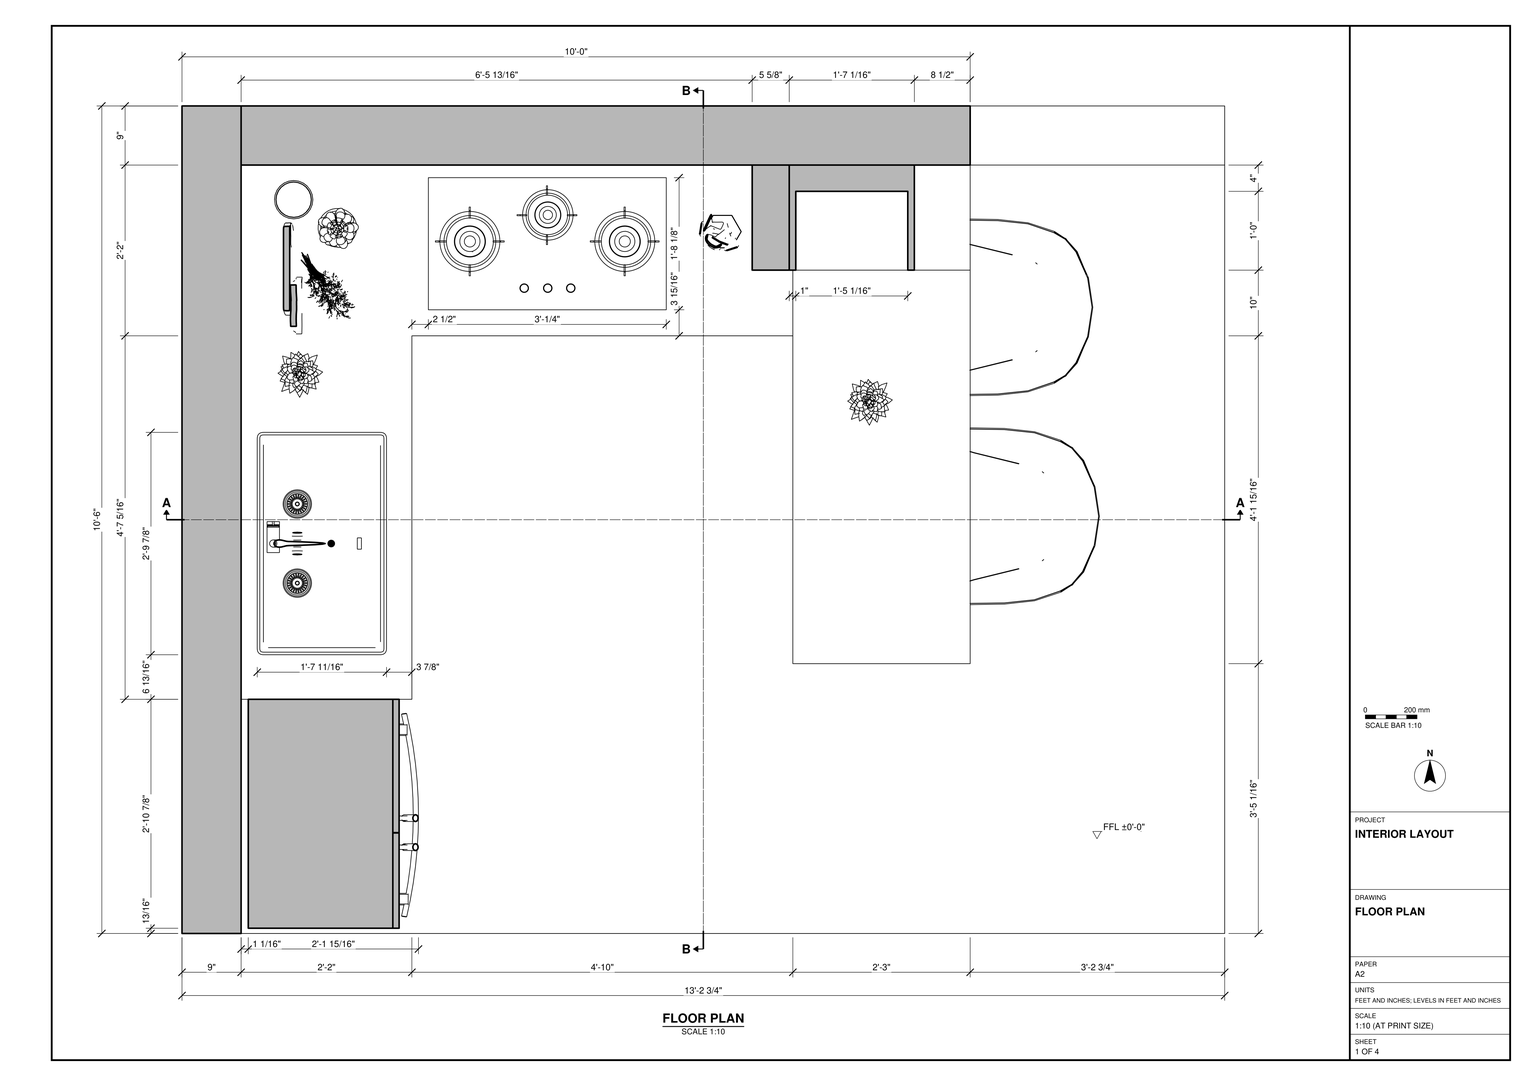
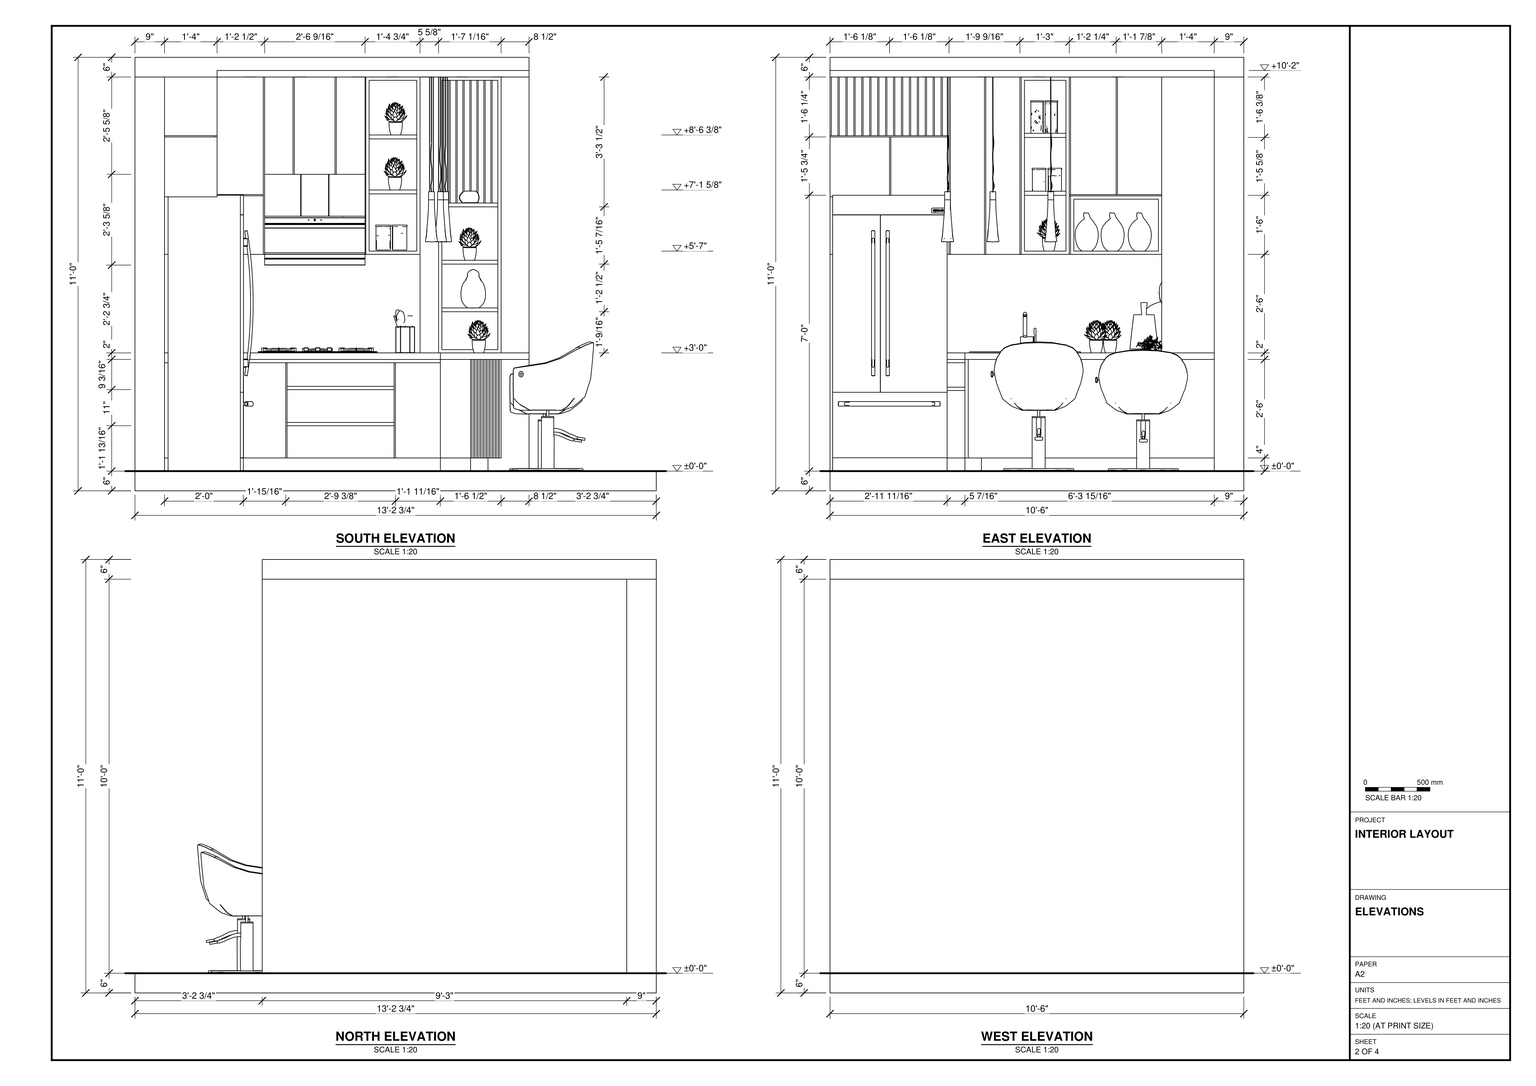
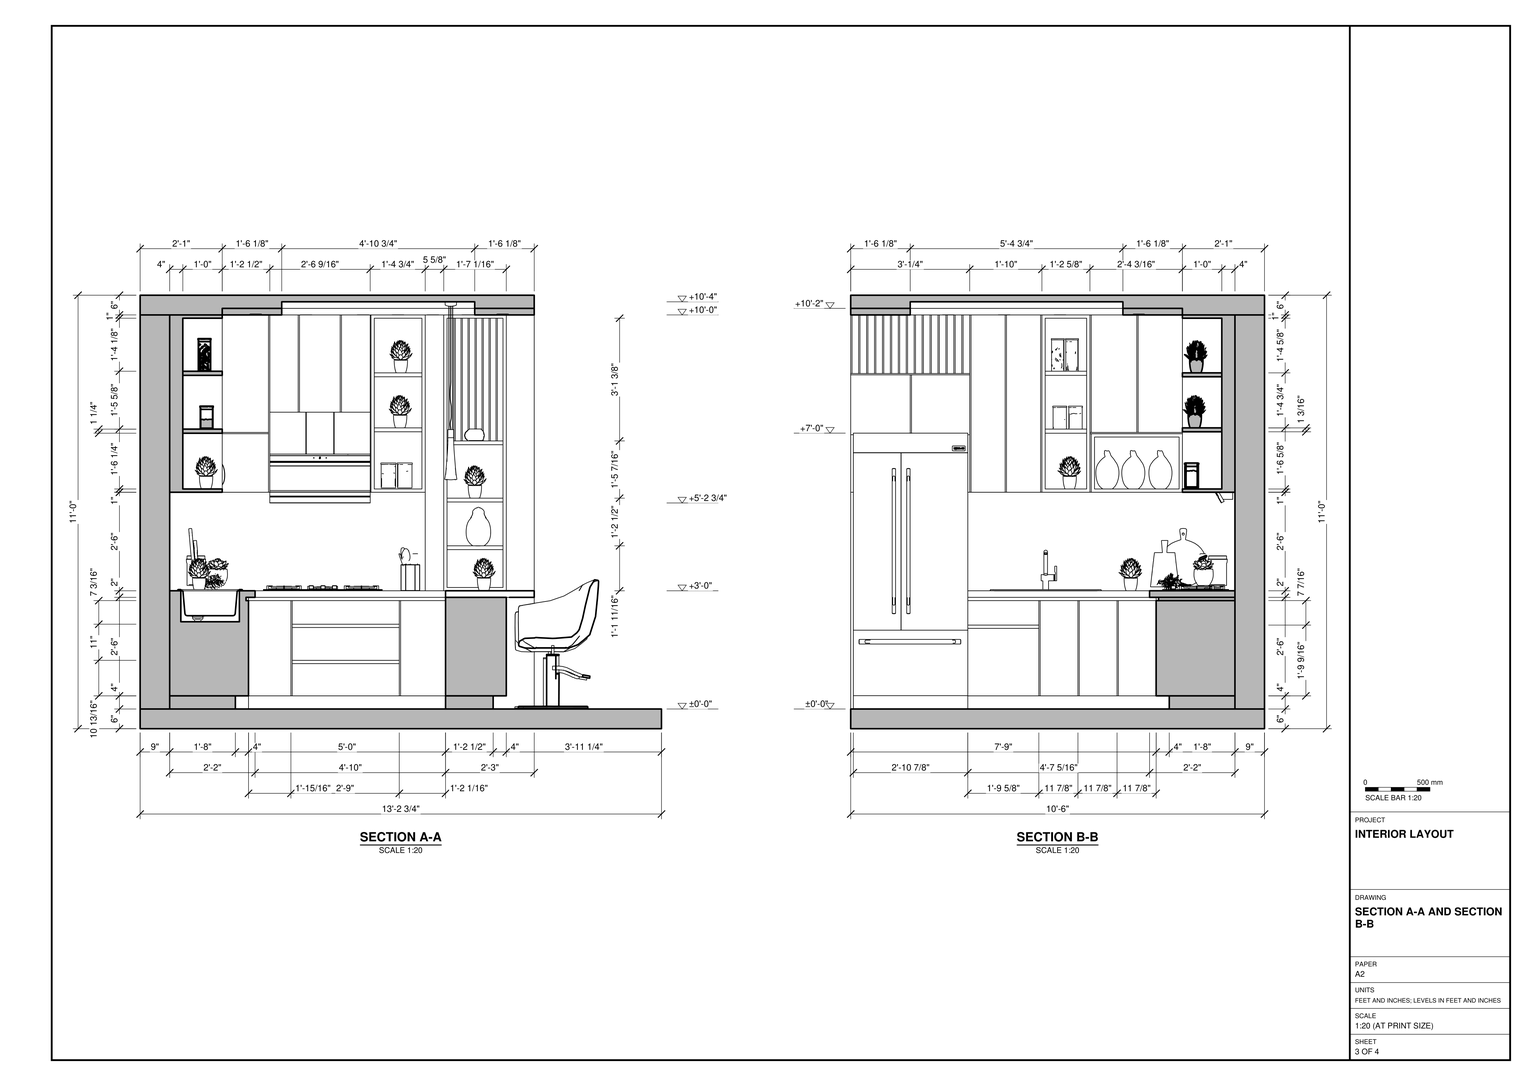
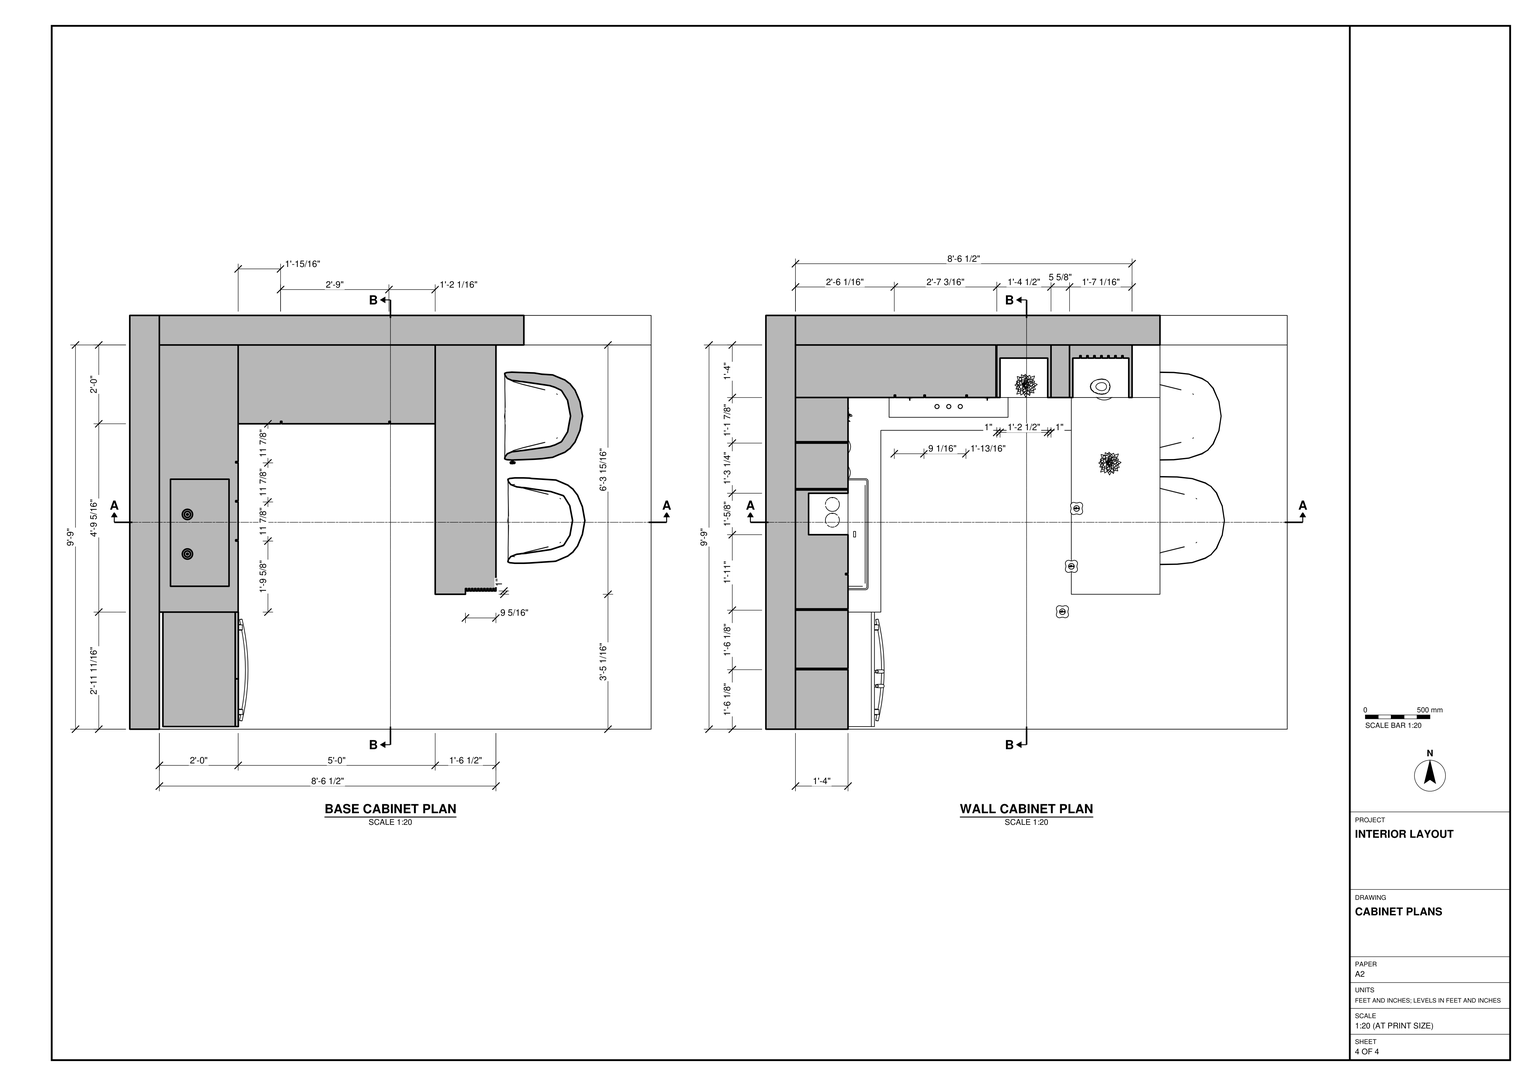
Build the kitchen interior in SketchUp from task_files/diagram_01.pdf. Work in feet and inches. The overall model measures 13'-2 3/4" along X, 10'-6" along Y and 11'-0" along Z. Set the finished floor at ±0'-0". Model the floor slab, the 9" thick north and west walls, and the stepped ceiling slab shown in section. The floor extends east beyond the end of the north wall to accommodate the seating.

Lay out the worktop along the two walls, with the sink and tap on the west run, the refrigerator at its south end, and the cooktop beneath the hood on the north run. Use the elevations and sections to set out the recessed plinths, base cabinet doors, drawer stack, upper cupboards, open shelves and vertically slatted panels. Match the shelf divisions around the hood and above the peninsula rather than treating the upper storage as a continuous bank of doors.

Project the peninsula south from the north run, leaving the working aisle between it and the sink. Place the two seats along its east edge and the pendant lights above it as drawn. Decor and loose items, including plants, vessels, utensils, lights and appliances, may be any suitable library components. Keep the walls, slabs and each furniture or joinery piece in separate groups or components, and use components for repeated parts. Save one SketchUp model as output_files/fitted_kitchen_with_a_seating_peninsula.skp.

# SketchUp Ruby script. Lengths in inches.
U = 1.inch
M = Sketchup.active_model
def pt(a) = Geom::Point3d.new(a.map { |v| v * U })
def face(e, loops, mat)
  f = e.add_face(loops[0].map { |a| pt(a) })
  loops[1..].each { |l| e.add_face(l.map { |a| pt(a) }).erase! }
  f.material = f.back_material = mat if mat
  f
end
# faces: each face lists its corners as indices into pts; further lists are holes
def faces(e, pts, list, mat = nil) = list.each { |f| face(e, (f[0].is_a?(Array) ? f : [f]).map { |l| l.map { |i| pts[i] } }, mat) }
# xy, xz, yz: faces in a plane at the given z, y or x. An outline is a flat list of corners, or four numbers for a rectangle; further outlines are holes
def ring(l) = l.size == 4 ? [[l[0], l[1]], [l[2], l[1]], [l[2], l[3]], [l[0], l[3]]] : l.each_slice(2).to_a
def flat(e, list, mat, &to3) = list.each { |f| face(e, (f[0].is_a?(Array) ? f : [f]).map { |l| ring(l).map { |u, v| to3.(u, v) } }, mat) }
def xy(e, z, list, mat = nil) = flat(e, list, mat) { |x, y| [x, y, z] }
def xz(e, y, list, mat = nil) = flat(e, list, mat) { |x, z| [x, y, z] }
def yz(e, x, list, mat = nil) = flat(e, list, mat) { |y, z| [x, y, z] }
def lines(e, pts, list) = list.each { |a, b| e.add_line(pt(pts[a]), pt(pts[b])) }
# prism: a flat outline (further loops are holes) pulled along v
def prism(e, loops, v, mat = nil)
  f = face(e, loops, mat); d = Geom::Vector3d.new(v.map { |x| x * U })
  f.pushpull(f.normal.samedirection?(d) ? d.length : -d.length)
end
def box(e, o, s, mat = nil) = prism(e, [[o, [o[0] + s[0], o[1], o[2]], [o[0] + s[0], o[1] + s[1], o[2]], [o[0], o[1] + s[1], o[2]]]], [0, 0, s[2]], mat)
def at(x, y, z, deg = 0) = Geom::Transformation.translation(pt([x, y, z])) * Geom::Transformation.rotation(ORIGIN, Z_AXIS, deg.degrees)
def axes(o, x, y, z) = Geom::Transformation.new([*x, 0, *y, 0, *z, 0, *pt(o).to_a, 1])
def part(name) = M.definitions.add(name)
# library, detail: a bought-in or finely detailed component or shape, given as its bounding box
def library(name, o, s) = part(name).tap { |d| box(d.entities, o, s) }
def detail(e, o, s) = box(e.add_group.entities, o, s)
def put(e, d, t, mat = nil) = e.add_instance(d, t).tap { |i| i.material = mat if mat }
def group(e, t, mat = nil) = e.add_group.tap { |g| g.transformation = t; g.material = mat if mat }.entities
root = M.entities
M.materials.add("Brush Stainles Steel").color = [21, 26, 31]
M.materials.add("Emissive").color = [220, 226, 183]
M.materials.add("Generic").color = [116, 116, 83]
M.materials.add("Generic\#1").color = [166, 178, 158]
M.materials.add("Marble White 100cm").color = [222, 222, 222]
M.materials.add("Material60").color = [0, 0, 8]
M.materials.add("[Color_I06]1").color = [12, 0, 204]
M.materials.add("stainless-steel2").color = [0, 0, 0]
c1 = library("Utensils",[0,-0.54,-0.24],[6.34,6.28,13.37])
c2 = library("ACCESS \#103",[-1.07,0,-1.17],[14.88,24.44,20.18])
c3 = library("kitchen utensils",[105.2,54.39,67.32],[65.26,45.04,45.46])
c4 = library("Tall kitchen cabinet",[0,0.54,0],[34.86,25.91,84])
c5 = library("Sink",[0,0,0],[33.86,19.69,21.73])
c6 = library("Bosch Stove",[0,0,0],[36.22,20.12,1.38])
c7 = part("-   0   +")
prism(c7.entities,[[[0.21,0.4375,-0.06],[0.46,0.4375,-0.06],[0.5,0.39,-0.06],[0.45,0.35,-0.06],[0.2,0.35,-0.06],[0.16,0.39,-0.06]]],[0,0,0.2],"[Color_I06]1")
prism(c7.entities,[[[2.39,0.79,-0.06],[2.65,0.79,-0.06],[2.6875,0.74,-0.06],[2.64,0.69,-0.06],[2.38,0.69,-0.06],[2.34,0.74,-0.06]]],[0,0,0.2],"[Color_I06]1")
prism(c7.entities,[[[2.33,0.09,-0.06],[2.59,0.09,-0.06],[2.625,0.05,-0.06],[2.58,0,-0.06],[2.32,0,-0.06],[2.28,0.05,-0.06]]],[0,0,0.2],"[Color_I06]1")
prism(c7.entities,[[[4.61,0.43,-0.06],[4.67,0.43,-0.06],[4.7,0.39,-0.06],[4.66,0.35,-0.06],[4.6,0.35,-0.06],[4.57,0.39,-0.06]]],[0,0,0.2],"[Color_I06]1")
prism(c7.entities,[[[4.82,0.35,-0.06],[4.75,0.35,-0.06],[4.72,0.39,-0.06],[4.76,0.43,-0.06],[4.82,0.43,-0.06],[4.86,0.39,-0.06]]],[0,0,0.2],"[Color_I06]1")
prism(c7.entities,[[[4.67,0.35,-0.06],[4.71,0.38,-0.06],[4.75,0.35,-0.06],[4.74,0.29,-0.06],[4.7,0.25,-0.06],[4.66,0.29,-0.06]]],[0,0,0.2],"[Color_I06]1")
prism(c7.entities,[[[4.68,0.5,-0.06],[4.72,0.54,-0.06],[4.76,0.5,-0.06],[4.75,0.4375,-0.06],[4.71,0.4,-0.06],[4.68,0.4375,-0.06]]],[0,0,0.2],"[Color_I06]1")
xy(c7.entities,-0.06,[[2.27,0.06,2.23,0.1,2.25,0.35,2.3,0.39,2.35,0.35,2.32,0.1],[2.64,0.06,2.59,0.1,2.62,0.35,2.67,0.39,2.71,0.35,2.6875,0.1],[2.3,0.39,2.26,0.4375,2.28,0.68,2.33,0.73,2.375,0.68,2.36,0.4375],[2.67,0.39,2.625,0.4375,2.65,0.68,2.7,0.73,2.74,0.68,2.72,0.4375]],"[Color_I06]1")
xy(c7.entities,0.14,[[2.27,0.06,2.32,0.1,2.35,0.35,2.3,0.39,2.25,0.35,2.23,0.1],[2.64,0.06,2.6875,0.1,2.71,0.35,2.67,0.39,2.62,0.35,2.59,0.1],[2.3,0.39,2.36,0.4375,2.375,0.68,2.33,0.73,2.28,0.68,2.26,0.4375],[2.67,0.39,2.72,0.4375,2.74,0.68,2.7,0.73,2.65,0.68,2.625,0.4375]],"[Color_I06]1")
p = [[2.23,0.1,-0.06],[2.27,0.06,-0.06],[2.27,0.06,0.14],[2.23,0.1,0.14],[2.25,0.35,-0.06],[2.25,0.35,0.14],
  [2.32,0.1,-0.06],[2.35,0.35,-0.06],[2.35,0.35,0.14],[2.32,0.1,0.14],[2.64,0.06,-0.06],[2.6875,0.1,-0.06],
  [2.6875,0.1,0.14],[2.64,0.06,0.14],[2.59,0.1,-0.06],[2.59,0.1,0.14],[2.62,0.35,-0.06],[2.62,0.35,0.14],
  [2.71,0.35,-0.06],[2.71,0.35,0.14],[2.3,0.39,-0.06],[2.3,0.39,0.14],[2.67,0.39,-0.06],[2.67,0.39,0.14],
  [2.36,0.4375,-0.06],[2.36,0.4375,0.14],[2.26,0.4375,-0.06],[2.26,0.4375,0.14],[2.28,0.68,-0.06],[2.28,0.68,0.14],
  [2.375,0.68,-0.06],[2.375,0.68,0.14],[2.625,0.4375,-0.06],[2.625,0.4375,0.14],[2.65,0.68,-0.06],[2.65,0.68,0.14],
  [2.72,0.4375,-0.06],[2.74,0.68,-0.06],[2.74,0.68,0.14],[2.72,0.4375,0.14],[2.33,0.73,-0.06],[2.33,0.73,0.14],
  [2.7,0.73,-0.06],[2.7,0.73,0.14]]
faces(c7.entities,p,[[0,1,2,3],[4,0,3,5],[6,7,8,9],[1,6,9,2],[10,11,12,13],[14,10,13,15],[16,14,15,17],[11,18,19,12],
  [20,4,5,21],[7,20,21,8],[22,16,17,23],[18,22,23,19],[20,24,25,21],[26,20,21,27],[28,26,27,29],[24,30,31,25],
  [32,22,23,33],[34,32,33,35],[36,37,38,39],[22,36,39,23],[40,28,29,41],[30,40,41,31],[42,34,35,43],[37,42,43,38]],"[Color_I06]1")
c8 = part("komin dół\#1")
prism(c8.entities,[[[9.06,9.76,0],[9.06,9.84,0],[9.92,9.84,0],[9.92,-0.08,0],[-0.08,-0.08,0],[-0.08,9.84,0],[0.79,9.84,0],[0.79,9.76,0],[0.08,9.76,0],[0.08,0.08,0],[9.76,0.08,0],[9.76,9.76,0]]],[0,0,18.125],"stainless-steel2")
c9 = part("komin")
put(c9.entities,c8,at(0,0,0),"Brush Stainles Steel")
c10 = part("korpus")
prism(c10.entities,[[[0,0,17.125],[0,13.78,17.125],[0,13.78,0],[0,9.89,0]]],[19.69,0,0],"stainless-steel2")
c11 = part("panel przód")
yz(c11.entities,0,[[11.02,0,9.65,2.39,9.82,2.49,11.19,0.1],[9.45,2.73,1.57,16.37,1.75,16.47,2.63,14.93,8.34,5.04,8.73,4.36,9.62,2.83],[1.38,16.71,0,19.09,0.17,19.19,1.55,16.81]],"Material60")
yz(c11.entities,0,[[11.19,0.1,9.82,2.49,9.99,2.58,8.9,4.46,8.73,4.36,8.34,5.04,2.63,14.93,2.8,15.03,1.72,16.9,1.55,16.81,0.17,19.19,1.19,19.78,12.22,0.6875]],"stainless-steel2")
yz(c11.entities,35.43,[[11.02,0,11.19,0.1,9.82,2.49,9.65,2.39],[9.45,2.73,9.62,2.83,8.73,4.36,8.34,5.04,2.63,14.93,1.75,16.47,1.57,16.37],[1.38,16.71,1.55,16.81,0.17,19.19,0,19.09]],"Material60")
yz(c11.entities,35.43,[[11.19,0.1,12.22,0.6875,1.19,19.78,0.17,19.19,1.55,16.81,1.72,16.9,2.8,15.03,2.63,14.93,8.34,5.04,8.73,4.36,8.9,4.46,9.99,2.58,9.82,2.49]],"stainless-steel2")
p = [[0,9.65,2.39],[0,11.02,0],[35.43,11.02,0],[35.43,9.65,2.39],[0,11.19,0.1],[35.43,11.19,0.1],
  [0,9.82,2.49],[35.43,9.82,2.49],[0,12.22,0.6875],[35.43,12.22,0.6875],[0,1.19,19.78],[35.43,1.19,19.78],
  [0,9.99,2.58],[35.43,9.99,2.58],[0,8.9,4.46],[35.43,8.9,4.46],[0,1.57,16.37],[0,9.45,2.73],
  [35.43,9.45,2.73],[35.43,1.57,16.37],[0,9.62,2.83],[35.43,9.62,2.83],[0,8.73,4.36],[35.43,8.73,4.36],
  [0,8.34,5.04],[35.43,8.34,5.04],[0,2.63,14.93],[35.43,2.63,14.93],[0,1.75,16.47],[35.43,1.75,16.47],
  [0,2.8,15.03],[35.43,2.8,15.03],[0,1.72,16.9],[35.43,1.72,16.9],[0,0,19.09],[0,1.38,16.71],
  [35.43,1.38,16.71],[35.43,0,19.09],[0,1.55,16.81],[35.43,1.55,16.81],[0,0.17,19.19],[35.43,0.17,19.19]]
faces(c11.entities,p,[[0,1,2,3],[1,4,5,2],[4,6,7,5],[6,0,3,7],[16,17,18,19],[17,20,21,18],[20,22,23,21],[22,24,25,23],
  [24,26,27,25],[26,28,29,27],[28,16,19,29],[34,35,36,37],[35,38,39,36],[38,40,41,39],[40,34,37,41]],"Material60")
faces(c11.entities,p,[[4,8,9,5],[8,10,11,9],[12,6,7,13],[14,12,13,15],[22,14,15,23],[30,26,27,31],[32,30,31,33],[38,32,33,39],
  [10,40,41,11]],"stainless-steel2")
c12 = part("BERG Spring 90")
p = [[27.56,1.88,18.59],[27.56,1.19,19.78]]
lines(c12.entities,p,[[0,1]])
put(c12.entities,c9,at(12.8,5.82,18.59))
put(c12.entities,c10,at(7.875,1.88,1.46))
put(c12.entities,c11,at(0,0,0))
c13 = part("BERG+Spring+90")
put(c13.entities,c7,axes([14.86,0.79,17.53],[0.97787,0,0],[0,-0.48894,0.84686],[0,-0.84686,-0.48894]))
put(c13.entities,c12,axes([0,0,0],[0.97787,0,0],[0,0.97787,0],[0,0,0.97787]))
c14 = library("Queen Mary The Styling Chair",[-14.34,-10.7,0],[28.08,24.6,32.26])
c15 = library("Potted Plant 50-23",[-3.4,-3.5,0],[6.8,7,9.93])
c16 = library("Interior Props 221 031",[-3.74,-3.52,-0.04],[7.48,7.03,11.78])
c17 = library("Bathroom Fixture 02 22-64",[-3.05,-2.36,0],[6.1,4.72,3.64])
c18 = library("Concra 152 061",[-1.85,-1.85,-54.21],[3.7,3.7,54.21])
c19 = library("Tlon Light 1950 Ceiling 152 010",[-38.39,-38.39,-3.78],[76.78,76.78,3.41])
xy(root,-6,[[0,0,158.75,126]])
xy(root,0,[[0,0,9,126],[9,0,158.75,0,158.75,117,107.5,117,107.5,46.08,102.21,46.08,102.21,41.08,93,41.08,93,97,29,97,29,35.66,9,35.66],[9,35.66,29,35.66,29,97,33,97,33,117,9,117],[93,41.08,102.21,41.08,102.21,46.08,107.5,46.08,107.5,117,33,117,33,97,93,97],[93,41.08,93,117,107.5,117,107.5,46.08,102.21,46.08,102.21,41.08],
  [33,97,93,117],[9,117,120,126],[120,117,158.75,126]])
xy(root,4,[[9,35.66,9,117,33,117,33,97,29,97,29,35.66],[29,35.66,33,57.28],[93,41.08,93,117,107.5,117,107.5,46.08,102.21,46.08,102.21,41.08],[102.61,42.08,102.61,42.83,102.21,42.83,102.21,46.08,107.5,46.08,107.5,42.08,107.25,42.08,107.25,42.83,106.85,42.83,106.85,42.08,106.33,42.08,106.33,42.83,105.93,42.83,105.93,42.08,105.4,42.08,105.4,42.83,105,42.83,105,42.08,104.47,42.08,104.47,42.83,104.07,42.83,104.07,42.08,103.54,42.08,103.54,42.83,103.14,42.83,103.14,42.08],[107.5,42.08,107.5,117,111.5,117,111.5,42.08,110.97,42.08,110.97,42.83,110.57,42.83,110.57,42.08,110.04,42.08,110.04,42.83,109.64,42.83,109.64,42.08,109.11,42.08,109.11,42.83,108.71,42.83,108.71,42.08,108.18,42.08,108.18,42.83,107.78,42.83,107.78,42.08],
  [29,57.28,32.25,57.68],[29,57.68,33,69.1875],[29,69.1875,32.25,69.59],[29,69.59,33,81.09],[29,81.09,32.25,81.49],
  [29,81.49,33,97],[33,93,45.91,97],[46.3125,93,78.91,97],[79.3125,93,93,97],[45.91,93.75,46.3125,97],
  [78.91,93.75,79.3125,97],[33,97,93,117]])
xy(root,13.8125,[[46.3125,93,78.91,93.75]],"Generic")
xy(root,14.8125,[[46.3125,93,78.91,93.75]],"Generic")
xy(root,24.55,[[32.25,35.66,33,57.28]],"Generic")
xy(root,24.8125,[[46.3125,93,78.91,93.75]],"Generic")
xy(root,25.55,[[32.25,35.66,33,57.28]],"Generic")
xy(root,25.8125,[[46.3125,93,78.91,93.75]],"Generic")
xy(root,26.5625,[[12.4,43.52,30.22,76.125]])
xy(root,33,[[33,93.75,93,117]])
xy(root,33,[[32.25,35.66,33,57.28],[32.25,57.68,33,69.1875],[32.25,69.59,33,81.09],[32.25,81.49,33,93],[33,93,45.91,93.75],
  [46.3125,93,78.91,93.75],[79.3125,93,93,93.75]],"Generic")
xy(root,34,[[93,41.08,93,117,111.5,117,111.5,42.08,110.97,42.08,110.97,42.83,110.57,42.83,110.57,42.08,110.04,42.08,110.04,42.83,109.64,42.83,109.64,42.08,109.11,42.08,109.11,42.83,108.71,42.83,108.71,42.08,108.18,42.08,108.18,42.83,107.78,42.83,107.78,42.08,107.25,42.08,107.25,42.83,106.85,42.83,106.85,42.08,106.33,42.08,106.33,42.83,105.93,42.83,105.93,42.08,105.4,42.08,105.4,42.83,105,42.83,105,42.08,104.47,42.08,104.47,42.83,104.07,42.83,104.07,42.08,103.54,42.08,103.54,42.83,103.14,42.83,103.14,42.08,102.61,42.08,102.61,42.83,102.21,42.83,102.21,41.08],[33,93.75,93,117]])
xy(root,34,[[32.25,91,33,93]],"Generic")
xy(root,34,[[32.25,35.66,35,91],[102.21,41.08,102.21,41.58,112.5,41.58,112.5,117,120,117,120,41.08],[33,91,93,93.75]],"Marble White 100cm")
xy(root,36,[[86.81,101,92.45,117],[92.45,101,93,117],[93,101,111.5,117],[111.5,101,120,117]])
xy(root,36,[[[9,35.66,35,35.66,35,91,93,91,93,101,86.81,101,86.81,117,9,117],[12.4,43.52,30.22,76.125]],[93,41.08,120,101]],"Marble White 100cm")
xy(root,37,[[93.45,101,110.5,113]],"Generic")
xy(root,48.53,[[93.45,112,110.5,113]],"Emissive")
xy(root,48.53,[[93.45,101,110.5,112]],"Generic")
xy(root,49.69,[[93.45,101,110.5,113]],"Generic")
xy(root,63.03,[[93.45,112,110.5,113]],"Emissive")
xy(root,63.03,[[93.45,101,110.5,112]],"Generic")
xy(root,64.19,[[93.45,101,110.5,113]],"Generic")
xy(root,66,[[9,36.64,9,117,39.49,117,39.49,116,10,116,10,36.64],[70.3,116,86.81,117]],"Emissive")
xy(root,66,[[9,36.24,24.25,36.64],[10,36.64,10,116,39.49,116,39.49,101.75,39.09,101.75,39.09,101,25,101,25,47.43,24.25,47.43,24.25,47.03,25,47.03,25,36.64],[70.3,101,86.81,116],[70.0625,101.75,70.3,117]],"Generic")
xy(root,67,[[71.3,101,85.81,113]])
xy(root,67,[[13,59.22,25,71.84],[13,74.24,25,100]],"Generic")
xy(root,80.47,[[93.45,112,110.5,113]],"Emissive")
xy(root,80.47,[[93.45,101,110.5,112]],"Generic")
xy(root,81.63,[[93.45,101,110.5,113],[95.58,113,95.98,113.75],[97.71,113,98.11,113.75],[99.84,113,100.24,113.75],[101.98,113,102.375,113.75],
  [104.11,113,104.51,113.75],[106.24,113,106.64,113.75],[108.37,113,108.77,113.75]],"Generic")
xy(root,82.82,[[13,74.24,14,100]],"Emissive")
xy(root,82.82,[[14,74.24,25,100]],"Generic")
xy(root,83.52,[[9,0,25,18.12],[9,18.12,24.25,18.51],[9,18.51,24.25,18.52],[9,18.52,25,36.24]])
xy(root,83.82,[[9,73.24,25,87.12],[9,87.12,25,101]])
xy(root,83.84,[[9,72.84,25,73.24],[9,73.24,25,101]])
xy(root,83.98,[[13,59.22,14,71.84]],"Emissive")
xy(root,83.98,[[14,59.22,25,71.84]],"Generic")
xy(root,84.22,[[9,72.84,25,73.24],[9,73.24,25,87.12],[9,87.12,25,87.52],[9,87.52,25,101]])
xy(root,84.41,[[71.3,112,85.81,113]],"Emissive")
xy(root,84.41,[[71.3,101,85.81,112]],"Generic")
xy(root,85.23,[[13,59.22,25,71.84]],"Generic")
xy(root,85.61,[[71.3,101,85.81,113]],"Generic")
xy(root,90.375,[[39.49,101,39.49,117,70.0625,117,70.0625,101,61.3125,101,61.3125,101.75,60.91,101.75,60.91,101,48.53,101,48.53,101.75,48.13,101.75,48.13,101]])
xy(root,101.16,[[71.3,112,85.81,113]],"Emissive")
xy(root,101.16,[[71.3,101,85.81,112]],"Generic")
xy(root,101.6,[[13,59.22,14,71.84]],"Emissive")
xy(root,101.6,[[14,59.22,25,71.84]],"Generic")
xy(root,101.76,[[9,0,24.25,18.12],[9,18.12,24.25,18.52],[9,18.52,24.25,36.24]])
xy(root,101.76,[[24.25,0,25,18.12],[24.25,18.52,25,36.24]],"Generic")
xy(root,102.16,[[9,0,24.25,18.12],[24.25,0,25,0.4],[9,18.12,24.25,36.24]])
xy(root,102.16,[[24.25,0.4,25,2.42],[24.25,2.82,25,4.83],[24.25,5.23,25,7.25],[24.25,7.65,25,9.66],[24.25,10.0625,25,12.08],
  [24.25,12.48,25,14.49],[24.25,14.89,25,16.91],[24.25,17.31,25,18.12],[24.25,18.12,25,19.33],[24.25,19.73,25,21.74],
  [24.25,22.14,25,24.16],[24.25,24.56,25,26.57],[24.25,26.97,25,28.99],[24.25,29.39,25,31.4],[24.25,31.8,25,33.82],
  [24.25,34.22,25,36.24]],"Generic")
xy(root,102.36,[[71.3,101,85.81,113]],"Generic")
xy(root,102.86,[[13,59.22,25,71.84]],"Generic")
xy(root,119,[[13,59.22,14,71.84],[71.3,112,85.81,113],[93.45,112.13,93.45,113,95.58,113,95.58,113.75,95.98,113.75,95.98,113,97.71,113,97.71,113.75,98.11,113.75,98.11,113,99.84,113,99.84,113.75,100.24,113.75,100.24,113,101.98,113,101.98,113.75,102.375,113.75,102.375,113,104.11,113,104.11,113.75,104.51,113.75,104.51,113,106.24,113,106.24,113.75,106.64,113.75,106.64,113,108.37,113,108.37,113.75,108.77,113.75,108.77,113,110.5,113,110.5,112.13]],"Emissive")
xy(root,119,[[14,59.22,25,71.84],[71.3,101,85.81,112],[93.45,101,110.5,112.13]],"Generic")
xy(root,120,[[0,0,9,126],[9,0,9,36.24,25,36.24,25,34.22,24.25,34.22,24.25,33.82,25,33.82,25,31.8,24.25,31.8,24.25,31.4,25,31.4,25,29.39,24.25,29.39,24.25,28.99,25,28.99,25,26.97,24.25,26.97,24.25,26.57,25,26.57,25,24.56,24.25,24.56,24.25,24.16,25,24.16,25,22.14,24.25,22.14,24.25,21.74,25,21.74,25,19.73,24.25,19.73,24.25,19.33,25,19.33,25,17.31,24.25,17.31,24.25,16.91,25,16.91,25,14.89,24.25,14.89,24.25,14.49,25,14.49,25,12.48,24.25,12.48,24.25,12.08,25,12.08,25,10.0625,24.25,10.0625,24.25,9.66,25,9.66,25,7.65,24.25,7.65,24.25,7.25,25,7.25,25,5.23,24.25,5.23,24.25,4.83,25,4.83,25,2.82,24.25,2.82,24.25,2.42,25,2.42,25,0],[[25,0,25,101,111.5,101,111.5,117,120,117,120,0],[43.12,18.12,101.88,82.88]],[9,36.24,24.25,36.64],[9,36.64,25,47.03],
  [9,47.03,24.25,47.43],[9,47.43,25,57.82],[9,57.82,25,58.22],[9,58.22,25,72.84],[9,72.84,25,73.24],
  [9,73.24,25,87.12],[9,87.12,25,87.52],[9,87.52,25,101],[9,101,25,117],[9,101,25,117],
  [25,101,25,117,70.0625,117,70.0625,101,61.3125,101,61.3125,101.75,60.91,101.75,60.91,101,48.53,101,48.53,101.75,48.13,101.75,48.13,101,39.49,101,39.49,101.75,39.09,101.75,39.09,101],[70.3,101,86.81,117],[86.81,101,92.45,117],[92.45,101,111.5,117],[70.0625,101.75,70.0625,117,9,117,9,126,120,126,120,117,70.3,117,70.3,101.75]])
xy(root,120,[[24.25,2.42,25,2.82],[24.25,4.83,25,5.23],[24.25,7.25,25,7.65],[24.25,9.66,25,10.0625],[24.25,12.08,25,12.48],
  [24.25,14.49,25,14.89],[24.25,16.91,25,17.31],[24.25,19.33,25,19.73],[24.25,21.74,25,22.14],[24.25,24.16,25,24.56],
  [24.25,26.57,25,26.97],[24.25,28.99,25,29.39],[24.25,31.4,25,31.8],[24.25,33.82,25,34.22],[24.25,36.24,25,36.64],
  [24.25,47.03,25,47.43],[39.09,101,39.49,101.75],[48.13,101,48.53,101.75],[60.91,101,61.3125,101.75],[70.0625,101,70.3,101.75]],"Generic")
xy(root,122,[[[25,0,120,0,120,117,111.5,117,111.5,101,25,101],[43.12,18.12,101.88,82.88]]])
xy(root,124,[[43.12,18.12,101.88,82.88]])
xy(root,126,[[0,0,120,126]])
xz(root,0,[[0,-6,158.75,0],[0,0,9,120],[9,83.52,25,101.76],[9,101.76,24.25,102.16],[9,102.16,25,120],
  [0,120,25,120,25,122,120,122,120,126,0,126],[25,120,120,122]])
xz(root,2.42,[[24.25,102.16,25,120]],"Generic")
xz(root,2.82,[[24.25,102.16,25,120]],"Generic")
xz(root,4.83,[[24.25,102.16,25,120]],"Generic")
xz(root,5.23,[[24.25,102.16,25,120]],"Generic")
xz(root,7.25,[[24.25,102.16,25,120]],"Generic")
xz(root,7.65,[[24.25,102.16,25,120]],"Generic")
xz(root,9.66,[[24.25,102.16,25,120]],"Generic")
xz(root,10.0625,[[24.25,102.16,25,120]],"Generic")
xz(root,12.08,[[24.25,102.16,25,120]],"Generic")
xz(root,12.48,[[24.25,102.16,25,120]],"Generic")
xz(root,14.49,[[24.25,102.16,25,120]],"Generic")
xz(root,14.89,[[24.25,102.16,25,120]],"Generic")
xz(root,16.91,[[24.25,102.16,25,120]],"Generic")
xz(root,17.31,[[24.25,102.16,25,120]],"Generic")
xz(root,18.12,[[9,83.52,24.25,101.76],[43.12,120,101.88,122]])
xz(root,18.12,[[43.12,122,101.88,124]],"Emissive")
xz(root,18.12,[[24.25,83.52,25,101.76]],"Generic")
xz(root,18.52,[[9,83.52,24.25,101.76]])
xz(root,18.52,[[24.25,83.52,25,101.76]],"Generic")
xz(root,19.33,[[24.25,102.16,25,120]],"Generic")
xz(root,19.73,[[24.25,102.16,25,120]],"Generic")
xz(root,21.74,[[24.25,102.16,25,120]],"Generic")
xz(root,22.14,[[24.25,102.16,25,120]],"Generic")
xz(root,24.16,[[24.25,102.16,25,120]],"Generic")
xz(root,24.56,[[24.25,102.16,25,120]],"Generic")
xz(root,26.57,[[24.25,102.16,25,120]],"Generic")
xz(root,26.97,[[24.25,102.16,25,120]],"Generic")
xz(root,28.99,[[24.25,102.16,25,120]],"Generic")
xz(root,29.39,[[24.25,102.16,25,120]],"Generic")
xz(root,31.4,[[24.25,102.16,25,120]],"Generic")
xz(root,31.8,[[24.25,102.16,25,120]],"Generic")
xz(root,33.82,[[24.25,102.16,25,120]],"Generic")
xz(root,34.22,[[24.25,102.16,25,120]],"Generic")
xz(root,35.66,[[9,0,29,4],[9,4,33,4,33,24.55,32.25,24.55,32.25,25.55,33,25.55,33,33,9,33]])
xz(root,35.66,[[9,33,32.25,33,32.25,34,35,34,35,36,9,36]],"Marble White 100cm")
xz(root,36.24,[[9,66,24.25,83.52],[9,83.52,24.25,101.76],[9,101.76,24.25,102.16],[9,102.16,24.25,120]])
xz(root,36.24,[[24.25,83.52,25,101.76],[24.25,102.16,25,120]],"Generic")
xz(root,36.64,[[9,66,24.25,83.52],[9,83.52,24.25,101.76],[9,101.76,24.25,102.16],[9,102.16,24.25,120]])
xz(root,36.64,[[24.25,66,25,83.52],[24.25,83.52,25,101.76],[24.25,101.76,25,102.16],[24.25,102.16,25,120]],"Generic")
xz(root,41.08,[[93,0,102.21,4]])
xz(root,41.08,[[93,4,102.21,34],[93,34,120,36]],"Marble White 100cm")
xz(root,42.08,[[102.61,4,103.14,34],[103.54,4,104.07,34],[104.47,4,105,34],[105.4,4,105.93,34],[106.33,4,106.85,34],
  [107.25,4,107.78,34],[108.18,4,108.71,34],[109.11,4,109.64,34],[110.04,4,110.57,34],[110.97,4,111.5,34]],"Generic")
xz(root,42.83,[[102.21,4,102.61,34],[103.14,4,103.54,34],[104.07,4,104.47,34],[105,4,105.4,34],[105.93,4,106.33,34],
  [106.85,4,107.25,34],[107.78,4,108.18,34],[108.71,4,109.11,34],[109.64,4,110.04,34],[110.57,4,110.97,34]],"Generic")
xz(root,43.52,[[12.4,26.5625,30.22,36]])
xz(root,46.08,[[102.21,0,107.5,4]])
xz(root,47.03,[[24.25,66,25,120]],"Generic")
xz(root,47.43,[[24.25,66,25,120]],"Generic")
xz(root,57.28,[[32.25,4,33,24.55],[32.25,25.55,33,33]],"Generic")
xz(root,57.68,[[32.25,4,33,33]],"Generic")
xz(root,59.22,[[13,67,25,83.98],[13,83.98,25,85.23],[13,101.6,25,102.86]])
xz(root,59.22,[[13,85.23,25,101.6],[13,102.86,25,119]],"Generic")
xz(root,69.1875,[[32.25,4,33,33]],"Generic")
xz(root,69.59,[[32.25,4,33,33]],"Generic")
xz(root,71.84,[[13,83.98,25,85.23],[13,101.6,25,102.86]])
xz(root,71.84,[[13,67,25,83.98],[13,85.23,25,101.6],[13,102.86,25,119]],"Generic")
xz(root,72.84,[[9,83.84,25,84.22],[9,84.22,25,120]])
xz(root,73.24,[[9,83.82,25,83.84],[9,84.22,25,120]])
xz(root,74.24,[[13,67,25,82.82]])
xz(root,76.125,[[12.4,26.5625,30.22,36]])
xz(root,81.09,[[32.25,4,33,33]],"Generic")
xz(root,81.49,[[32.25,4,33,33]],"Generic")
xz(root,82.88,[[43.12,120,101.88,122]])
xz(root,82.88,[[43.12,122,101.88,124]],"Emissive")
xz(root,87.12,[[9,84.22,25,120]])
xz(root,87.52,[[9,84.22,25,120]])
xz(root,91,[[35,34,93,36]],"Marble White 100cm")
xz(root,93,[[33,4,45.91,33],[46.3125,4,78.91,13.8125],[79.3125,4,93,33],[46.3125,14.8125,78.91,24.8125],[46.3125,25.8125,78.91,33],
  [32.25,33,33,34]],"Generic")
xz(root,93.75,[[45.91,4,46.3125,33],[78.91,4,79.3125,33],[46.3125,13.8125,78.91,14.8125],[46.3125,24.8125,78.91,25.8125],[33,33,93,34]],"Generic")
xz(root,97,[[29,0,33,4],[33,0,93,4]])
xz(root,100,[[13,67,25,82.82]],"Generic")
xz(root,101,[[9,83.82,25,83.84],[9,83.84,25,84.22],[9,84.22,25,120],[25,120,39.09,122],[39.09,120,39.49,122],
  [39.49,120,48.13,122],[48.13,120,48.53,122],[48.53,120,60.91,122],[60.91,120,61.3125,122],[61.3125,120,70.0625,122],
  [70.0625,120,70.3,122],[70.3,120,86.81,122],[86.81,120,92.45,122],[92.45,120,111.5,122]])
xz(root,101,[[[92.45,36,111.5,120],[93.45,37,110.5,119]],[93.45,48.53,110.5,49.69],[93.45,63.03,110.5,64.19],[25,66,39.09,83.84],[[70.3,66,86.81,120],[71.3,67,85.81,119]],
  [93.45,80.47,110.5,81.63],[25,83.84,39.09,84.22],[71.3,84.41,85.81,85.61],[71.3,101.16,85.81,102.36]],"Generic")
xz(root,101,[[86.81,36,92.45,120],[25,84.22,39.09,120],[39.49,90.375,48.13,120],[48.53,90.375,60.91,120],[61.3125,90.375,70.0625,120]],"Generic\#1")
xz(root,101.75,[[39.09,66,39.49,120],[70.0625,66,70.3,120],[48.13,90.375,48.53,120],[60.91,90.375,61.3125,120]],"Generic")
xz(root,113,[[93.45,48.53,110.5,49.69],[93.45,63.03,110.5,64.19],[93.45,80.47,110.5,81.63],[71.3,84.41,85.81,85.61],[71.3,101.16,85.81,102.36]])
xz(root,113,[[93.45,37,110.5,48.53],[93.45,49.69,110.5,63.03],[93.45,64.19,110.5,80.47],[71.3,67,85.81,84.41],[93.45,81.63,95.58,119],
  [95.98,81.63,97.71,119],[98.11,81.63,99.84,119],[100.24,81.63,101.98,119],[102.375,81.63,104.11,119],[104.51,81.63,106.24,119],
  [106.64,81.63,108.37,119],[108.77,81.63,110.5,119],[71.3,85.61,85.81,101.16],[71.3,102.36,85.81,119]],"Generic")
xz(root,113.75,[[95.58,81.63,95.98,119],[97.71,81.63,98.11,119],[99.84,81.63,100.24,119],[101.98,81.63,102.375,119],[104.11,81.63,104.51,119],
  [106.24,81.63,106.64,119],[108.37,81.63,108.77,119]],"Generic")
xz(root,117,[[9,0,33,4],[33,0,93,4],[93,0,107.5,4],[107.5,0,120,0,120,34,111.5,34,111.5,4,107.5,4],[9,4,33,33],
  [33,4,93,33],[93,4,111.5,34],[9,33,33,36],[33,33,93,34],[33,34,93,36],
  [93,34,120,36],[86.81,36,92.45,120],[92.45,36,111.5,120],[111.5,36,120,120],[9,66,25,120],
  [25,66,39.49,66,39.49,90.375,70.0625,90.375,70.0625,120,25,120],[70.3,66,86.81,120],[111.5,120,120,122]])
xz(root,117,[[9,36,86.81,36,86.81,66,70.0625,66,70.0625,90.375,39.49,90.375,39.49,66,9,66]],"Marble White 100cm")
xz(root,126,[[0,-6,158.75,0],[0,0,9,120],[9,0,120,120],[0,120,120,126]])
yz(root,0,[[0,-6,126,0],[0,0,126,120],[0,120,126,126]])
yz(root,9,[[35.66,0,117,4],[117,0,126,120],[35.66,4,117,33],[35.66,33,117,36],[0,66,36.24,83.52],
  [36.24,66,36.64,120],[36.64,66,47.03,120],[47.03,66,47.43,120],[47.43,66,57.82,120],[57.82,66,58.22,120],
  [58.22,66,72.84,120],[72.84,66,73.24,83.84],[73.24,66,101,83.82],[101,66,117,120],[0,83.52,18.12,101.76],
  [18.12,83.52,18.52,101.76],[18.52,83.52,36.24,101.76],[73.24,83.82,101,83.84],[72.84,83.84,73.24,84.22],[73.24,83.84,101,84.22],
  [72.84,84.22,73.24,120],[73.24,84.22,87.12,120],[87.12,84.22,87.52,120],[87.52,84.22,101,120],[0,101.76,36.24,102.16],
  [0,102.16,36.24,120]])
yz(root,9,[[0,0,35.66,0,35.66,36,117,36,117,66,0,66]],"Marble White 100cm")
yz(root,12.4,[[43.52,26.5625,76.125,36]])
yz(root,13,[[59.22,83.98,71.84,85.23],[59.22,101.6,71.84,102.86]])
yz(root,13,[[59.22,67,71.84,83.98],[74.24,67,100,82.82],[59.22,85.23,71.84,101.6],[59.22,102.86,71.84,119]],"Generic")
yz(root,24.25,[[36.24,66,36.64,120],[47.03,66,47.43,120],[18.12,83.52,18.52,101.76],[0,101.76,36.24,102.16],[2.42,102.16,2.82,120],
  [4.83,102.16,5.23,120],[7.25,102.16,7.65,120],[9.66,102.16,10.0625,120],[12.08,102.16,12.48,120],[14.49,102.16,14.89,120],
  [16.91,102.16,17.31,120],[19.33,102.16,19.73,120],[21.74,102.16,22.14,120],[24.16,102.16,24.56,120],[26.57,102.16,26.97,120],
  [28.99,102.16,29.39,120],[31.4,102.16,31.8,120],[33.82,102.16,34.22,120]],"Generic")
yz(root,25,[[0,120,0.4,122],[0.4,120,2.42,122],[2.42,120,2.82,122],[2.82,120,4.83,122],[4.83,120,5.23,122],
  [5.23,120,7.25,122],[7.25,120,7.65,122],[7.65,120,9.66,122],[9.66,120,10.0625,122],[10.0625,120,12.08,122],
  [12.08,120,12.48,122],[12.48,120,14.49,122],[14.49,120,14.89,122],[14.89,120,16.91,122],[16.91,120,17.31,122],
  [17.31,120,19.33,122],[19.33,120,19.73,122],[19.73,120,21.74,122],[21.74,120,22.14,122],[22.14,120,24.16,122],
  [24.16,120,24.56,122],[24.56,120,26.57,122],[26.57,120,26.97,122],[26.97,120,28.99,122],[28.99,120,29.39,122],
  [29.39,120,31.4,122],[31.4,120,31.8,122],[31.8,120,33.82,122],[33.82,120,34.22,122],[34.22,120,36.24,122],
  [36.24,120,36.64,122],[36.64,120,47.03,122],[47.03,120,47.43,122],[47.43,120,57.82,122],[57.82,120,58.22,122],
  [58.22,120,72.84,122],[72.84,120,73.24,122],[73.24,120,87.12,122],[87.12,120,87.52,122],[87.52,120,101,122]])
yz(root,25,[[57.82,66,58.22,120],[[58.22,66,72.84,120],[59.22,67,71.84,119]],[72.84,66,73.24,83.84],[[73.24,66,101,83.82],[74.24,67,100,82.82]],[72.84,83.84,101,84.22],
  [59.22,83.98,71.84,85.23],[72.84,84.22,73.24,120],[87.12,84.22,87.52,120],[59.22,101.6,71.84,102.86],[0,102.16,0.4,120],
  [0.4,102.16,2.42,120],[2.82,102.16,4.83,120],[5.23,102.16,7.25,120],[7.65,102.16,9.66,120],[10.0625,102.16,12.08,120],
  [12.48,102.16,14.49,120],[14.89,102.16,16.91,120],[17.31,102.16,19.33,120],[19.73,102.16,21.74,120],[22.14,102.16,24.16,120],
  [24.56,102.16,26.57,120],[26.97,102.16,28.99,120],[29.39,102.16,31.4,120],[31.8,102.16,33.82,120],[34.22,102.16,36.24,120]],"Generic")
yz(root,25,[[36.64,66,47.03,120],[47.43,66,57.82,120],[0,83.52,18.12,101.76],[18.52,83.52,36.24,101.76],[73.24,84.22,87.12,120],
  [87.52,84.22,101,120]],"Generic\#1")
yz(root,29,[[35.66,0,97,4]])
yz(root,30.22,[[43.52,26.5625,76.125,36]])
yz(root,32.25,[[57.28,4,57.68,33],[69.1875,4,69.59,33],[81.09,4,81.49,33],[35.66,24.55,57.28,25.55],[35.66,33,93,34]],"Generic")
yz(root,33,[[97,0,117,4],[93,4,117,33],[93.75,33,117,34]])
yz(root,33,[[35.66,4,57.28,24.55],[57.68,4,69.1875,33],[69.59,4,81.09,33],[81.49,4,93,33],[35.66,25.55,57.28,33],
  [93,33,93.75,34]],"Generic")
yz(root,35,[[35.66,34,91,36]],"Marble White 100cm")
yz(root,39.09,[[101,66,101.75,83.84],[101,83.84,101.75,84.22],[101,84.22,101.75,90.375],[101,90.375,101.75,120]],"Generic")
yz(root,39.49,[[101.75,66,117,90.375],[101,90.375,101.75,120]],"Generic")
yz(root,43.12,[[18.12,120,82.88,122]])
yz(root,43.12,[[18.12,122,82.88,124]],"Emissive")
yz(root,45.91,[[93,4,93.75,33]],"Generic")
yz(root,46.3125,[[93,4,93.75,13.8125],[93,14.8125,93.75,24.8125],[93,25.8125,93.75,33]],"Generic")
yz(root,48.13,[[101,90.375,101.75,120]],"Generic")
yz(root,48.53,[[101,90.375,101.75,120]],"Generic")
yz(root,60.91,[[101,90.375,101.75,120]],"Generic")
yz(root,61.3125,[[101,90.375,101.75,120]],"Generic")
yz(root,70.0625,[[101.75,66,117,90.375],[101.75,90.375,117,120]])
yz(root,70.0625,[[101,90.375,101.75,120]],"Generic")
yz(root,70.3,[[101.75,66,117,120]])
yz(root,70.3,[[101,66,101.75,120]],"Generic")
yz(root,71.3,[[101,84.41,113,85.61],[101,101.16,113,102.36]])
yz(root,71.3,[[101,67,113,84.41],[101,85.61,113,101.16],[101,102.36,113,119]],"Generic")
yz(root,78.91,[[93,4,93.75,13.8125],[93,14.8125,93.75,24.8125],[93,25.8125,93.75,33]],"Generic")
yz(root,79.3125,[[93,4,93.75,33]],"Generic")
yz(root,85.81,[[101,84.41,113,85.61],[101,101.16,113,102.36]])
yz(root,85.81,[[101,67,113,84.41],[101,85.61,113,101.16],[101,102.36,113,119]],"Generic")
yz(root,86.81,[[101,36,117,66],[101,66,117,120]])
yz(root,92.45,[[101,36,117,120]])
yz(root,93,[[41.08,0,97,4],[97,0,117,4],[41.08,4,41.08,34,93.75,34,93.75,33,93,33,93,4],[93,4,117,33],[93.75,33,117,34],
  [41.08,34,91,36],[91,34,117,36]])
yz(root,93.45,[[101,48.53,113,49.69],[101,63.03,113,64.19],[101,80.47,113,81.63]])
yz(root,93.45,[[101,37,113,48.53],[101,49.69,113,63.03],[101,64.19,113,80.47],[101,81.63,113,119]],"Generic")
yz(root,95.58,[[113,81.63,113.75,119]],"Generic")
yz(root,95.98,[[113,81.63,113.75,119]],"Generic")
yz(root,97.71,[[113,81.63,113.75,119]],"Generic")
yz(root,98.11,[[113,81.63,113.75,119]],"Generic")
yz(root,99.84,[[113,81.63,113.75,119]],"Generic")
yz(root,100.24,[[113,81.63,113.75,119]],"Generic")
yz(root,101.88,[[18.12,120,82.88,122]])
yz(root,101.88,[[18.12,122,82.88,124]],"Emissive")
yz(root,101.98,[[113,81.63,113.75,119]],"Generic")
yz(root,102.21,[[41.08,0,46.08,4],[41.08,4,42.83,34]])
yz(root,102.375,[[113,81.63,113.75,119]],"Generic")
yz(root,102.61,[[42.08,4,42.83,34]],"Generic")
yz(root,103.14,[[42.08,4,42.83,34]],"Generic")
yz(root,103.54,[[42.08,4,42.83,34]],"Generic")
yz(root,104.07,[[42.08,4,42.83,34]],"Generic")
yz(root,104.11,[[113,81.63,113.75,119]],"Generic")
yz(root,104.47,[[42.08,4,42.83,34]],"Generic")
yz(root,104.51,[[113,81.63,113.75,119]],"Generic")
yz(root,105,[[42.08,4,42.83,34]],"Generic")
yz(root,105.4,[[42.08,4,42.83,34]],"Generic")
yz(root,105.93,[[42.08,4,42.83,34]],"Generic")
yz(root,106.24,[[113,81.63,113.75,119]],"Generic")
yz(root,106.33,[[42.08,4,42.83,34]],"Generic")
yz(root,106.64,[[113,81.63,113.75,119]],"Generic")
yz(root,106.85,[[42.08,4,42.83,34]],"Generic")
yz(root,107.25,[[42.08,4,42.83,34]],"Generic")
yz(root,107.5,[[46.08,0,117,4]])
yz(root,107.78,[[42.08,4,42.83,34]],"Generic")
yz(root,108.18,[[42.08,4,42.83,34]],"Generic")
yz(root,108.37,[[113,81.63,113.75,119]],"Generic")
yz(root,108.71,[[42.08,4,42.83,34]],"Generic")
yz(root,108.77,[[113,81.63,113.75,119]],"Generic")
yz(root,109.11,[[42.08,4,42.83,34]],"Generic")
yz(root,109.64,[[42.08,4,42.83,34]],"Generic")
yz(root,110.04,[[42.08,4,42.83,34]],"Generic")
yz(root,110.5,[[101,48.53,113,49.69],[101,63.03,113,64.19],[101,80.47,113,81.63]])
yz(root,110.5,[[101,37,113,48.53],[101,49.69,113,63.03],[101,64.19,113,80.47],[101,81.63,113,119]],"Generic")
yz(root,110.57,[[42.08,4,42.83,34]],"Generic")
yz(root,110.97,[[42.08,4,42.83,34]],"Generic")
yz(root,111.5,[[101,120,117,122]])
yz(root,111.5,[[42.08,4,117,34],[101,36,117,120]],"Generic")
yz(root,120,[[117,0,126,120],[41.08,34,117,36],[0,120,117,122],[117,120,126,120,126,126,0,126,0,122,117,122]])
yz(root,158.75,[[0,-6,126,0]])
p = [[9,18.51,83.52],[9,18.51,83.47],[9,18.52,101.78],[9,18.52,101.76],[9,101,83.84],[9,101.12,83.84],
  [33,91,36],[33,91,34]]
lines(root,p,[[0,1],[2,3],[4,5],[6,7]])
put(root,c1,at(78.8125,103.95,36))
put(root,c2,at(14.07,91.29,36))
put(root,c3,at(-87.58,6.6875,0))
put(root,c4,at(36.54,0.8,0,90),"Generic")
put(root,c5,at(31.14,42.44,26.64,90))
put(root,c6,at(37.51,94.96,36.2))
put(root,c13,axes([39.49,104.52,62.73],[0.88246,0,0],[0,0.77,0],[0,0,0.77]))
put(root,c14,axes([125.77,62.72,0],[0,-1,0],[1,0,0],[0,0,1.22]))
put(root,c15,at(104.75,80.88,36))
put(root,c15,at(101.98,106.1,64.19))
put(root,c15,at(79.43,105.09,102.36))
put(root,c15,at(79.22,104.62,85.61))
put(root,c15,at(18.01,85.13,36))
put(root,c15,at(20.125,66.53,67))
put(root,c16,at(103,103.76,49.69))
put(root,c16,at(21.07,94.32,67))
put(root,c16,at(22.05,86.05,67))
put(root,c16,at(21.97,78.16,67))
put(root,c17,at(101.79,104.32,81.63))
put(root,c14,axes([124.77,94.54,0],[0,-1,0],[1,0,0],[0,0,1.14677]))
put(root,c18,at(94.6,67.22,124))
put(root,c18,at(93.03,49.59,124))
put(root,c18,at(90.29,35.78,124))
put(root,c19,axes([110.39,12.72,120.18],[0.0473,0,0],[0,0.0473,0],[0,0,0.0473]))
put(root,c19,axes([110.39,29.72,120.18],[0.0473,0,0],[0,0.0473,0],[0,0,0.0473]))
put(root,c19,axes([110.39,46.72,120.18],[0.0473,0,0],[0,0.0473,0],[0,0,0.0473]))
put(root,c19,axes([110.39,63.72,120.18],[0.0473,0,0],[0,0.0473,0],[0,0,0.0473]))
put(root,c19,axes([35.21,29.72,120.18],[0.0473,0,0],[0,0.0473,0],[0,0,0.0473]))
put(root,c19,axes([35.21,46.72,120.18],[0.0473,0,0],[0,0.0473,0],[0,0,0.0473]))
put(root,c19,axes([35.21,63.72,120.18],[0.0473,0,0],[0,0.0473,0],[0,0,0.0473]))
put(root,c19,axes([35.21,12.72,120.18],[0.0473,0,0],[0,0.0473,0],[0,0,0.0473]))
put(root,c19,axes([35.21,87.81,120.18],[0.0473,0,0],[0,0.0473,0],[0,0,0.0473]))
put(root,c19,axes([110.39,87.72,120.18],[0.0473,0,0],[0,0.0473,0],[0,0,0.0473]))
put(root,c19,axes([99.77,87.72,120.18],[0.0473,0,0],[0,0.0473,0],[0,0,0.0473]))
put(root,c19,axes([89.14,87.72,120.18],[0.0473,0,0],[0,0.0473,0],[0,0,0.0473]))
put(root,c19,axes([78.52,87.72,120.18],[0.0473,0,0],[0,0.0473,0],[0,0,0.0473]))
put(root,c19,axes([67.89,87.72,120.18],[0.0473,0,0],[0,0.0473,0],[0,0,0.0473]))
put(root,c19,axes([50.52,87.72,120.18],[0.0473,0,0],[0,0.0473,0],[0,0,0.0473]))
